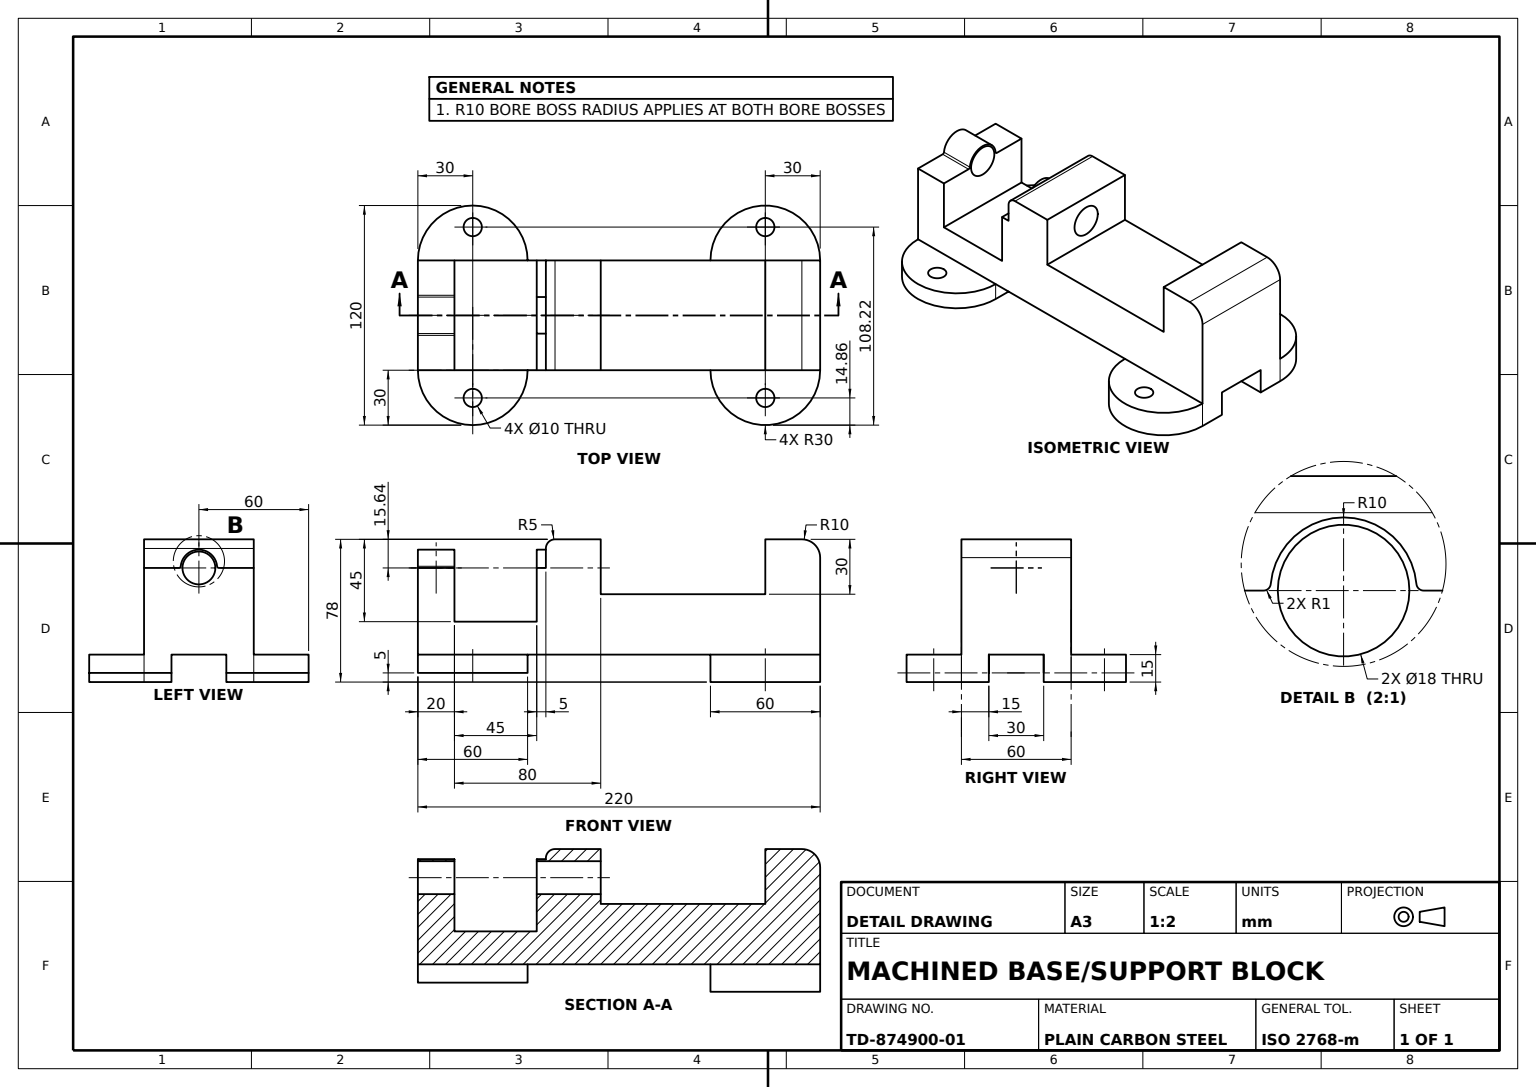
solid
v1 (90,-15,-83.223644)
v2 (90,0,-83.223644)
e1 v1 v2 LINE
v3 (90,0,-73.223644)
e2 v2 v3 CIRCLE(AX(P(90,0,-78.223644),D(0,1,0),D(0,0,1)),5)
v4 (90,-15,-73.223644)
e3 v4 v3 LINE
e4 v1 v4 CIRCLE(AX(P(90,-15,-78.223644),D(0,1,0),D(0,0,1)),5)
face CYL(AX(P(90,-15,-78.223644),D(0,1,0),D(0,0,1)),5) rev [e1 e2 -e3 -e4]
e5 v4 v1 CIRCLE(AX(P(90,-15,-78.223644),D(0,1,0),D(0,0,1)),5)
v5 (120,-15,-45)
v6 (120,-15,-60)
e6 v5 v6 LINE
v7 (60,-15,-45)
e7 v5 v7 LINE
v8 (60,-15,-60)
e8 v7 v8 LINE
e9 v8 v6 CIRCLE(AX(P(90,-15,-60),D(0,-1,0),D(0,0,-1)),30)
face PLANE(AX(P(120,-15,-45),D(0,1,0),D(0,0,-1))) rev [e5 e4] [-e6 e7 e8 e9]
v9 (-70,-10,10.138678)
v10 (-70,-10,20.138678)
e10 v9 v10 CIRCLE(AX(P(-70,-10,15.138678),D(0,1,0),D(0,0,1)),5)
e11 v10 v9 CIRCLE(AX(P(-70,-10,15.138678),D(0,1,0),D(0,0,1)),5)
v11 (-70,-10,30)
v12 (-40,-10,0)
e12 v11 v12 CIRCLE(AX(P(-70,-10,0),D(0,1,0),D(0,0,1)),30)
v13 (-100,-10,0)
e13 v13 v11 CIRCLE(AX(P(-70,-10,0),D(0,1,0),D(0,0,1)),30)
v14 (-100,-10,-15)
e14 v14 v13 LINE
v15 (-40,-10,-15)
e15 v15 v14 LINE
e16 v15 v12 LINE
face PLANE(AX(P(-100,-10,-15),D(0,1,0),D(0,0,1))) rev [e10 e11] [-e12 -e13 -e14 -e15 e16]
v16 (-35,18,-60)
v17 (-80,18,-60)
e17 v16 v17 LINE
v18 (-80,18,0)
e18 v18 v17 LINE
v19 (-35,18,0)
e19 v18 v19 LINE
e20 v16 v19 LINE
face PLANE(AX(P(0,18,0),D(0,1,0),D(0,0,1))) [e17 -e18 e19 -e20]
v20 (-70,0,20.138678)
e21 v10 v20 LINE
v21 (-70,0,10.138678)
e22 v20 v21 CIRCLE(AX(P(-70,0,15.138678),D(0,1,0),D(0,0,1)),5)
e23 v9 v21 LINE
face CYL(AX(P(-70,-15,15.138678),D(0,1,0),D(0,0,1)),5) rev [e21 e22 -e23 -e11]
v22 (-40,-10,-45)
v23 (-100,-10,-45)
e24 v22 v23 LINE
v24 (-40,0,-45)
e25 v24 v22 LINE
v25 (-100,0,-45)
e26 v25 v24 LINE
e27 v23 v25 LINE
face PLANE(AX(P(0,0,-45),D(0,0,-1),D(1,0,0))) rev [-e24 -e25 -e26 -e27]
v26 (-70,-10,-73.223644)
v27 (-70,0,-73.223644)
e28 v26 v27 LINE
v28 (-70,-10,-83.223644)
e29 v28 v26 CIRCLE(AX(P(-70,-10,-78.223644),D(0,1,0),D(0,0,1)),5)
v29 (-70,0,-83.223644)
e30 v28 v29 LINE
e31 v29 v27 CIRCLE(AX(P(-70,0,-78.223644),D(0,1,0),D(0,0,1)),5)
face CYL(AX(P(-70,-15,-78.223644),D(0,1,0),D(0,0,1)),5) rev [-e28 -e29 e30 e31]
v30 (-25,63,-60)
v31 (-25,63,0)
e32 v30 v31 LINE
v32 (0,63,0)
e33 v31 v32 LINE
v33 (0,63,-60)
e34 v33 v32 LINE
e35 v33 v30 LINE
face PLANE(AX(P(0,63,0),D(0,-1,0),D(0,0,-1))) rev [e32 e33 -e34 e35]
v34 (90,0,10.138678)
v35 (90,0,20.138678)
e36 v34 v35 CIRCLE(AX(P(90,0,15.138678),D(0,1,0),D(0,0,1)),5)
v36 (90,-15,20.138678)
e37 v36 v35 LINE
v37 (90,-15,10.138678)
e38 v37 v36 CIRCLE(AX(P(90,-15,15.138678),D(0,1,0),D(0,0,1)),5)
e39 v37 v34 LINE
face CYL(AX(P(90,-15,15.138678),D(0,1,0),D(0,0,1)),5) rev [e36 -e37 -e38 e39]
v38 (0,33,-60)
v39 (0,33,0)
e40 v38 v39 LINE
e41 v38 v33 LINE
e42 v39 v32 LINE
v40 (0,47.357373,-39)
v41 (0,47.357373,-21)
e43 v40 v41 CIRCLE(AX(P(0,47.357373,-30),D(-1,0,0),D(0,0,1)),9)
e44 v41 v40 CIRCLE(AX(P(0,47.357373,-30),D(-1,0,0),D(0,0,1)),9)
face PLANE(AX(P(0,33,-60),D(-1,0,0),D(0,0,1))) rev [-e40 e41 e34 -e42] [e43 e44]
e45 v35 v34 CIRCLE(AX(P(90,0,15.138678),D(0,1,0),D(0,0,1)),5)
e46 v36 v37 CIRCLE(AX(P(90,-15,15.138678),D(0,1,0),D(0,0,1)),5)
face CYL(AX(P(90,-15,15.138678),D(0,1,0),D(0,0,1)),5) rev [e37 e45 -e39 -e46]
v42 (-100,-10,-60)
e47 v23 v42 LINE
v43 (-70,-10,-90)
e48 v42 v43 CIRCLE(AX(P(-70,-10,-60),D(0,-1,0),D(0,0,-1)),30)
v44 (-40,-10,-60)
e49 v43 v44 CIRCLE(AX(P(-70,-10,-60),D(0,-1,0),D(0,0,-1)),30)
e50 v22 v44 LINE
e51 v26 v28 CIRCLE(AX(P(-70,-10,-78.223644),D(0,1,0),D(0,0,1)),5)
face PLANE(AX(P(-100,-10,-45),D(0,1,0),D(0,0,-1))) rev [e47 e48 e49 -e50 e24] [e29 e51]
v45 (-40,0,-60)
e52 v45 v44 LINE
e53 v24 v45 LINE
face PLANE(AX(P(-40,-10,-45),D(-1,0,0),D(0,0,-1))) rev [-e52 -e53 e25 e50]
v46 (90,33,-60)
e54 v46 v38 LINE
v47 (90,33,0)
e55 v39 v47 LINE
e56 v46 v47 LINE
face PLANE(AX(P(0,33,0),D(0,1,0),D(0,0,1))) [e54 e40 e55 -e56]
v48 (-70,0,-90)
e57 v48 v45 CIRCLE(AX(P(-70,0,-60),D(0,-1,0),D(0,0,-1)),30)
e58 v43 v48 LINE
face CYL(AX(P(-70,-15,-60),D(0,1,0),D(0,0,-1)),30) [e57 e52 -e49 e58]
v49 (-30,47.357373,-20)
v50 (-30,47.357373,0)
e59 v49 v50 LINE
v51 (-30,58,0)
e60 v50 v51 LINE
v52 (-30,58,-60)
e61 v51 v52 LINE
v53 (-30,47.357373,-60)
e62 v53 v52 LINE
v54 (-30,47.357373,-40)
e63 v53 v54 LINE
e64 v49 v54 CIRCLE(AX(P(-30,47.357373,-30),D(-1,0,0),D(0,0,1)),10)
face PLANE(AX(P(-30,18,0),D(-1,0,0),D(0,0,1))) [e59 e60 e61 -e62 e63 -e64]
v55 (60,-15,-15)
v56 (60,-15,0)
e65 v55 v56 LINE
v57 (120,-15,-15)
e66 v57 v55 LINE
v58 (120,-15,0)
e67 v57 v58 LINE
e68 v56 v58 CIRCLE(AX(P(90,-15,0),D(0,1,0),D(0,0,1)),30)
face PLANE(AX(P(120,-15,-15),D(0,1,0),D(0,0,1))) rev [-e65 -e66 e67 -e68] [e38 e46]
v59 (110,63,0)
v60 (110,63,-60)
e69 v59 v60 LINE
v61 (120,53,0)
e70 v61 v59 CIRCLE(AX(P(110,53,0),D(0,0,1),D(-1,0,0)),10)
v62 (120,53,-60)
e71 v62 v61 LINE
e72 v60 v62 CIRCLE(AX(P(110,53,-60),D(0,0,-1),D(1,0,0)),10)
face CYL(AX(P(110,53,0),D(0,0,-1),D(-1,0,0)),10) [-e69 -e70 -e71 -e72]
v63 (60,0,-15)
e73 v55 v63 LINE
v64 (120,0,-15)
e74 v63 v64 LINE
e75 v64 v57 LINE
face PLANE(AX(P(0,0,-15),D(0,0,-1),D(-1,0,0))) [e73 e74 e75 e66]
e76 v21 v20 CIRCLE(AX(P(-70,0,15.138678),D(0,1,0),D(0,0,1)),5)
face CYL(AX(P(-70,-15,15.138678),D(0,1,0),D(0,0,1)),5) rev [e23 e76 -e21 -e10]
v65 (-100,47.357373,-19.045549)
v66 (-100,47.357373,0)
e77 v65 v66 LINE
v67 (-80,47.357373,0)
e78 v67 v66 LINE
v68 (-80,47.357373,-19.045549)
e79 v67 v68 LINE
e80 v68 v65 LINE
face PLANE(AX(P(-60,47.357373,0),D(0,-1,0),D(0,0,-1))) rev [e77 -e78 e79 e80]
v69 (-35,47.357373,-20)
e81 v69 v49 LINE
v70 (-35,47.357373,0)
e82 v69 v70 LINE
e83 v70 v50 LINE
face PLANE(AX(P(-35,47.357373,0),D(0,1,0),D(0,0,1))) [-e81 e82 e83 -e59]
v71 (120,0,-60)
v72 (60,0,-60)
e84 v71 v72 LINE
e85 v72 v71 CIRCLE(AX(P(90,0,-60),D(0,-1,0),D(-1,0,0)),30)
e86 v3 v2 CIRCLE(AX(P(90,0,-78.223644),D(0,1,0),D(0,0,1)),5)
face PLANE(AX(P(120,0,-90),D(0,-1,0),D(1,0,0))) rev [-e84 -e85] [-e2 -e86]
v73 (-40,0,0)
v74 (-100,0,0)
e87 v73 v74 LINE
v75 (-70,0,30)
e88 v74 v75 CIRCLE(AX(P(-70,0,0),D(0,1,0),D(0,0,1)),30)
e89 v75 v73 CIRCLE(AX(P(-70,0,0),D(0,1,0),D(0,0,1)),30)
face PLANE(AX(P(-40,0,30),D(0,-1,0),D(0,0,-1))) rev [e87 e88 e89] [-e76 -e22]
e90 v6 v71 LINE
e91 v8 v72 LINE
face CYL(AX(P(90,-30,-60),D(0,1,0),D(-1,0,0)),30) [-e90 -e9 e91 e85]
v76 (-100,0,-60)
e92 v76 v42 LINE
e93 v76 v48 CIRCLE(AX(P(-70,0,-60),D(0,-1,0),D(0,0,-1)),30)
face CYL(AX(P(-70,-15,-60),D(0,1,0),D(0,0,-1)),30) [-e92 e93 -e58 -e48]
e94 v31 v51 CIRCLE(AX(P(-25,58,0),D(0,0,1),D(-1,0,0)),5)
e95 v19 v70 LINE
e96 v18 v67 LINE
e97 v66 v74 LINE
v77 (60,0,0)
e98 v73 v77 LINE
v78 (120,0,0)
e99 v78 v77 LINE
e100 v61 v78 LINE
v79 (90,63,0)
e101 v79 v59 LINE
e102 v47 v79 LINE
face PLANE(AX(P(0,15,0),D(0,0,-1),D(-1,0,0))) rev [e42 -e33 e94 -e60 -e83 -e95 -e19 e96 e78 e97 -e87 e98 -e99 -e100 e70 -e101 -e102 -e55]
v80 (120,0,-45)
e103 v64 v80 LINE
e104 v80 v5 LINE
e105 v71 v62 LINE
e106 v58 v78 LINE
face PLANE(AX(P(120,0,0),D(-1,0,0),D(0,0,1))) rev [-e75 e103 e104 e6 e90 e105 e71 e100 -e106 -e67]
e107 v27 v29 CIRCLE(AX(P(-70,0,-78.223644),D(0,1,0),D(0,0,1)),5)
e108 v45 v76 LINE
face PLANE(AX(P(-40,0,-90),D(0,-1,0),D(0,0,1))) rev [-e31 -e107] [-e93 -e108 -e57]
v81 (60,0,-45)
e109 v7 v81 LINE
e110 v81 v72 LINE
face PLANE(AX(P(60,-15,-45),D(1,0,0),D(0,1,0))) rev [e109 e110 -e91 -e8]
e111 v52 v30 CIRCLE(AX(P(-25,58,-60),D(0,0,-1),D(1,0,0)),5)
face CYL(AX(P(-25,58,0),D(0,0,1),D(1,0,0)),5) [-e111 -e61 -e94 -e32]
e112 v81 v80 LINE
face PLANE(AX(P(0,0,-45),D(0,0,1),D(-1,0,0))) [-e7 -e104 -e112 -e109]
e113 v11 v75 LINE
e114 v73 v12 LINE
face CYL(AX(P(-70,-15,0),D(0,1,0),D(0,0,1)),30) [-e113 e12 -e114 -e89]
v82 (-35,47.357373,-21)
v83 (-35,47.357373,-39)
e115 v82 v83 CIRCLE(AX(P(-35,47.357373,-30),D(-1,0,0),D(0,0,1)),9)
e116 v83 v82 CIRCLE(AX(P(-35,47.357373,-30),D(-1,0,0),D(0,0,1)),9)
v84 (-35,47.357373,-60)
v85 (-35,47.357373,-40)
e117 v84 v85 LINE
e118 v84 v16 LINE
e119 v69 v85 CIRCLE(AX(P(-35,47.357373,-30),D(-1,0,0),D(0,0,1)),10)
face PLANE(AX(P(-35,0,0),D(-1,0,0),D(0,0,1))) [-e115 -e116] [-e117 e118 e20 e95 -e82 e119]
face CYL(AX(P(-70,-15,-78.223644),D(0,1,0),D(0,0,1)),5) rev [-e51 e28 e107 -e30]
v86 (90,63,-60)
e120 v46 v86 LINE
e121 v86 v79 LINE
face PLANE(AX(P(90,33,0),D(-1,0,0),D(0,0,1))) [-e120 e56 e102 -e121]
face CYL(AX(P(90,-15,-78.223644),D(0,1,0),D(0,0,1)),5) rev [-e5 e3 e86 -e1]
v87 (-80,48.266464,-39.958592)
v88 (-80,47.357373,-40.954451)
e122 v87 v88 CIRCLE(AX(P(-80,48.357373,-40.954451),D(1,0,0),D(0,0,-1)),1)
v89 (-100,47.357373,-40.954451)
e123 v89 v88 LINE
v90 (-100,48.266464,-39.958592)
e124 v89 v90 CIRCLE(AX(P(-100,48.357373,-40.954451),D(-1,0,0),D(0,0,-1)),1)
e125 v87 v90 LINE
face CYL(AX(P(-80,48.357373,-40.954451),D(-1,0,0),D(0,0,1)),1) rev [e122 -e123 e124 -e125]
e126 v40 v83 LINE
e127 v41 v82 LINE
face CYL(AX(P(44,47.357373,-30),D(-1,0,0),D(0,0,1)),9) rev [-e126 -e44 e127 e115]
v91 (-80,47.357373,-21)
v92 (-100,47.357373,-21)
e128 v91 v92 LINE
v93 (-80,47.357373,-39)
e129 v91 v93 CIRCLE(AX(P(-80,47.357373,-30),D(1,0,0),D(0,0,-1)),9)
v94 (-100,47.357373,-39)
e130 v93 v94 LINE
e131 v92 v94 CIRCLE(AX(P(-100,47.357373,-30),D(1,0,0),D(0,0,-1)),9)
face CYL(AX(P(44,47.357373,-30),D(-1,0,0),D(0,0,1)),9) rev [-e128 e129 e130 -e131]
v95 (-100,0,-15)
v96 (-40,0,-15)
e132 v95 v96 LINE
e133 v25 v95 LINE
e134 v72 v45 LINE
e135 v63 v77 LINE
e136 v96 v73 LINE
face PLANE(AX(P(0,0,0),D(0,1,0),D(0,0,1))) rev [-e132 -e133 e26 e53 -e134 -e110 e112 -e103 -e74 e135 -e98 -e136]
e137 v84 v53 LINE
e138 v85 v54 LINE
face PLANE(AX(P(-35,47.357373,0),D(0,1,0),D(0,0,1))) [-e137 e117 e138 -e63]
e139 v77 v78 CIRCLE(AX(P(90,0,0),D(0,1,0),D(-1,0,0)),30)
face PLANE(AX(P(120,0,30),D(0,-1,0),D(1,0,0))) rev [e99 e139] [-e45 -e36]
v97 (-100,48.266464,-20.041408)
v98 (-80,48.266464,-20.041408)
e140 v97 v98 LINE
e141 v98 v87 CIRCLE(AX(P(-80,47.357373,-30),D(-1,0,0),D(0,0,1)),10)
e142 v97 v90 CIRCLE(AX(P(-100,47.357373,-30),D(-1,0,0),D(0,0,1)),10)
face CYL(AX(P(-80,47.357373,-30),D(-1,0,0),D(0,0,1)),10) [e140 e141 e125 -e142]
e143 v93 v91 CIRCLE(AX(P(-80,47.357373,-30),D(1,0,0),D(0,0,-1)),9)
v99 (-80,47.357373,-60)
e144 v17 v99 LINE
e145 v99 v88 LINE
e146 v68 v98 CIRCLE(AX(P(-80,48.357373,-19.045549),D(1,0,0),D(0,0,-1)),1)
face PLANE(AX(P(-80,18,0),D(1,0,0),D(0,0,-1))) [-e129 -e143] [-e79 -e96 e18 e144 e145 -e122 -e141 -e146]
e147 v74 v13 LINE
face CYL(AX(P(-70,-15,0),D(0,1,0),D(0,0,1)),30) [e113 -e88 e147 e13]
e148 v96 v15 LINE
e149 v14 v95 LINE
face PLANE(AX(P(0,0,-15),D(0,0,1),D(1,0,0))) rev [e148 e15 e149 e132]
face CYL(AX(P(-35,47.357373,-30),D(1,0,0),D(0,0,-1)),10) [e81 e64 -e138 -e119]
e150 v94 v92 CIRCLE(AX(P(-100,47.357373,-30),D(1,0,0),D(0,0,-1)),9)
e151 v97 v65 CIRCLE(AX(P(-100,48.357373,-19.045549),D(-1,0,0),D(0,0,-1)),1)
v100 (-100,47.357373,-60)
e152 v89 v100 LINE
e153 v100 v76 LINE
face PLANE(AX(P(-100,15,-60),D(1,0,0),D(0,0,-1))) rev [e150 e131] [-e151 e142 -e124 e152 e153 e92 -e47 e27 e133 -e149 e14 -e147 -e97 -e77]
face CYL(AX(P(-80,48.357373,-19.045549),D(-1,0,0),D(0,0,1)),1) rev [e151 -e80 e146 -e140]
face CYL(AX(P(44,47.357373,-30),D(-1,0,0),D(0,0,1)),9) rev [-e150 -e130 e143 e128]
e154 v99 v100 LINE
face PLANE(AX(P(-60,47.357373,0),D(0,1,0),D(0,0,1))) [e154 -e152 e123 -e145]
face PLANE(AX(P(-40,-10,-15),D(-1,0,0),D(0,0,1))) rev [-e16 -e148 e136 e114]
e155 v60 v86 LINE
face PLANE(AX(P(0,63,0),D(0,-1,0),D(0,0,-1))) rev [e121 e101 e69 e155]
e156 v56 v77 LINE
face PLANE(AX(P(60,-15,-15),D(1,0,0),D(0,1,0))) rev [-e135 -e73 e65 e156]
face CYL(AX(P(44,47.357373,-30),D(-1,0,0),D(0,0,1)),9) rev [-e43 e126 e116 -e127]
face CYL(AX(P(90,-30,0),D(0,1,0),D(-1,0,0)),30) [e68 e106 -e139 -e156]
face PLANE(AX(P(100,15,-60),D(0,0,1),D(1,0,0))) rev [e120 -e155 e72 -e105 e84 e134 e108 -e153 -e154 -e144 -e17 -e118 e137 e62 e111 -e35 -e41 -e54]
